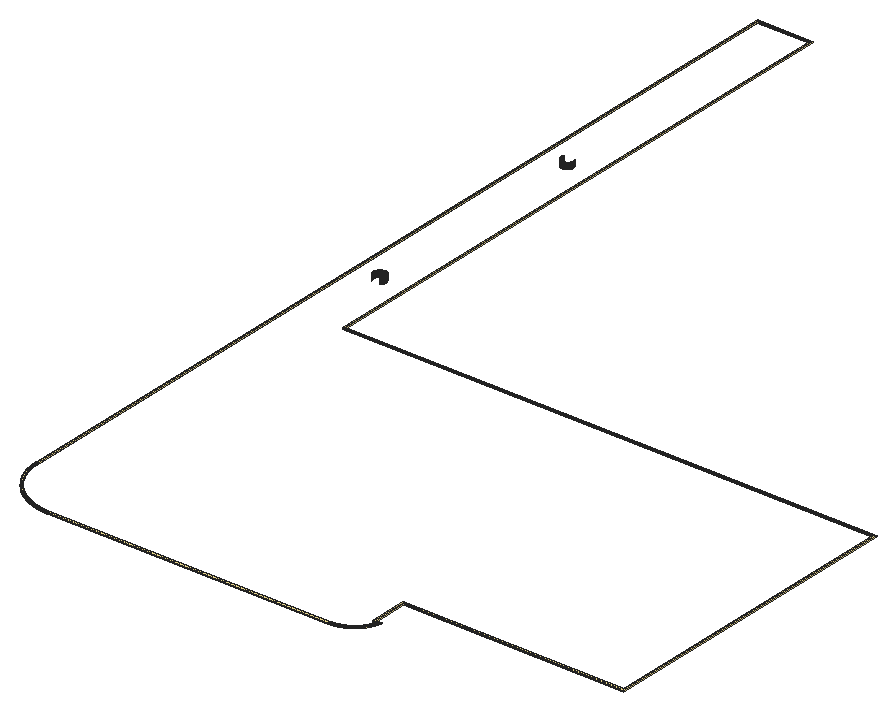
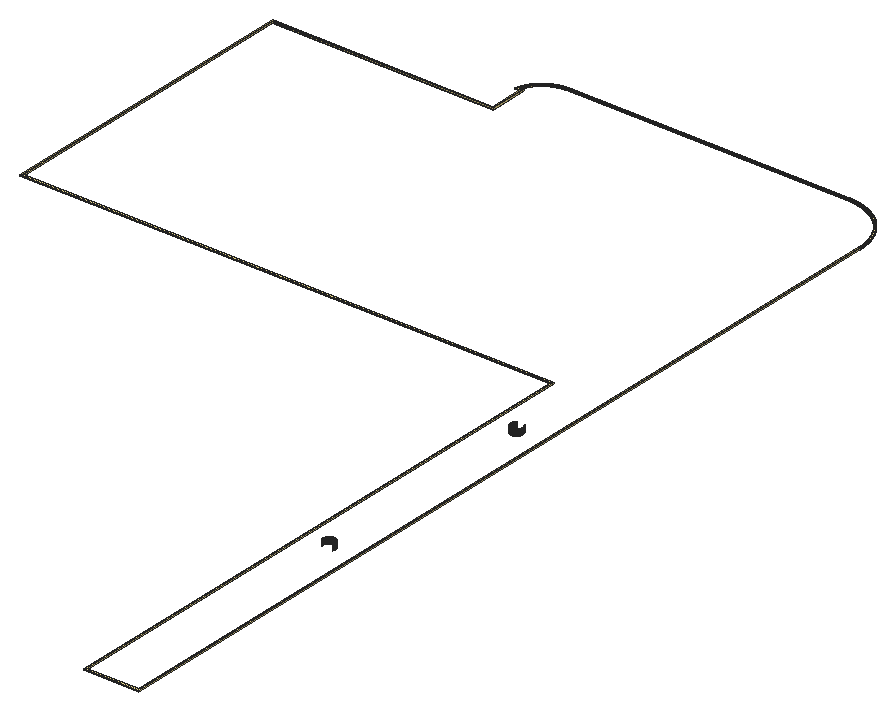
# SketchUp Ruby script. Lengths in inches.
U = 1.inch
M = Sketchup.active_model
def pt(a) = Geom::Point3d.new(a.map { |v| v * U })
def face(e, loops, mat)
  f = e.add_face(loops[0].map { |a| pt(a) })
  loops[1..].each { |l| e.add_face(l.map { |a| pt(a) }).erase! }
  f.material = f.back_material = mat if mat
  f
end
# faces: each face lists its corners as indices into pts; further lists are holes
def faces(e, pts, list, mat = nil) = list.each { |f| face(e, (f[0].is_a?(Array) ? f : [f]).map { |l| l.map { |i| pts[i] } }, mat) }
# xy, xz, yz: faces in a plane at the given z, y or x. An outline is a flat list of corners, or four numbers for a rectangle; further outlines are holes
def ring(l) = l.size == 4 ? [[l[0], l[1]], [l[2], l[1]], [l[2], l[3]], [l[0], l[3]]] : l.each_slice(2).to_a
def flat(e, list, mat, &to3) = list.each { |f| face(e, (f[0].is_a?(Array) ? f : [f]).map { |l| ring(l).map { |u, v| to3.(u, v) } }, mat) }
def xy(e, z, list, mat = nil) = flat(e, list, mat) { |x, y| [x, y, z] }
def xz(e, y, list, mat = nil) = flat(e, list, mat) { |x, z| [x, y, z] }
def yz(e, x, list, mat = nil) = flat(e, list, mat) { |y, z| [x, y, z] }
def lines(e, pts, list) = list.each { |a, b| e.add_line(pt(pts[a]), pt(pts[b])) }
# prism: a flat outline (further loops are holes) pulled along v
def prism(e, loops, v, mat = nil)
  f = face(e, loops, mat); d = Geom::Vector3d.new(v.map { |x| x * U })
  f.pushpull(f.normal.samedirection?(d) ? d.length : -d.length)
end
def box(e, o, s, mat = nil) = prism(e, [[o, [o[0] + s[0], o[1], o[2]], [o[0] + s[0], o[1] + s[1], o[2]], [o[0], o[1] + s[1], o[2]]]], [0, 0, s[2]], mat)
def at(x, y, z, deg = 0) = Geom::Transformation.translation(pt([x, y, z])) * Geom::Transformation.rotation(ORIGIN, Z_AXIS, deg.degrees)
def axes(o, x, y, z) = Geom::Transformation.new([*x, 0, *y, 0, *z, 0, *pt(o).to_a, 1])
def part(name) = M.definitions.add(name)
# library, detail: a bought-in or finely detailed component or shape, given as its bounding box
def library(name, o, s) = part(name).tap { |d| box(d.entities, o, s) }
def detail(e, o, s) = box(e.add_group.entities, o, s)
def put(e, d, t, mat = nil) = e.add_instance(d, t).tap { |i| i.material = mat if mat }
def group(e, t, mat = nil) = e.add_group.tap { |g| g.transformation = t; g.material = mat if mat }.entities
root = M.entities
M.materials.add("False Ceiling Light").color = [251, 231, 149]
xz(root,298.66,[[28.76,258,28.84,261],[29.16,258,29.24,261]])
xz(root,298.67,[[28.92,258,29,261],[29,258,29.08,261]])
xz(root,410.83,[[28.92,258,29,261],[29,258,29.08,261]])
xz(root,410.84,[[28.76,258,28.84,261],[29.16,258,29.24,261]])
yz(root,26,[[295.51,258,295.59,261],[295.59,258,295.67,261],[295.67,258,295.75,261],[295.75,258,295.82,261],[413.68,258,413.75,261],
  [413.75,258,413.83,261],[413.83,258,413.91,261],[413.91,258,413.99,261]])
yz(root,32,[[295.51,258,295.59,261],[295.59,258,295.67,261],[295.67,258,295.75,261],[295.75,258,295.82,261],[413.68,258,413.75,261],
  [413.75,258,413.83,261],[413.83,258,413.91,261],[413.91,258,413.99,261]])
p = [[26.99,293.4375,258],[26.93,293.49,258],[26.93,293.49,261],[26.99,293.4375,261],[31.07,293.49,258],[31.01,293.4375,258],
  [31.01,293.4375,261],[31.07,293.49,261],[26.88,293.55,258],[26.82,293.6,258],[26.82,293.6,261],[26.88,293.55,261],
  [31.12,293.55,258],[31.12,293.55,261],[31.18,293.6,258],[31.18,293.6,261],[26.77,293.66,258],[26.77,293.66,261],
  [31.23,293.66,258],[31.23,293.66,261],[26.72,293.72,258],[26.72,293.72,261],[26.67,293.78,258],[26.67,293.78,261],
  [31.28,293.72,258],[31.28,293.72,261],[31.33,293.78,258],[31.33,293.78,261],[26.62,293.84,258],[26.62,293.84,261],
  [26.57,293.9,258],[26.57,293.9,261],[31.38,293.84,258],[31.38,293.84,261],[31.43,293.9,258],[31.43,293.9,261],
  [26.53,293.97,258],[26.53,293.97,261],[31.47,293.97,258],[31.47,293.97,261],[26.48,294.03,258],[26.44,294.1,258],
  [26.44,294.1,261],[26.48,294.03,261],[31.52,294.03,258],[31.52,294.03,261],[31.56,294.1,258],[31.56,294.1,261],
  [26.4,294.17,258],[26.4,294.17,261],[31.6,294.17,258],[31.6,294.17,261],[26.36,294.24,258],[26.33,294.3,258],
  [26.33,294.3,261],[26.36,294.24,261],[31.64,294.24,258],[31.64,294.24,261],[31.67,294.3,258],[31.67,294.3,261],
  [26.29,294.375,258],[26.29,294.375,261],[31.71,294.375,258],[31.71,294.375,261],[26.26,294.45,258],[26.23,294.52,258],
  [26.23,294.52,261],[26.26,294.45,261],[31.74,294.45,258],[31.74,294.45,261],[31.77,294.52,258],[31.77,294.52,261],
  [26.2,294.59,258],[26.2,294.59,261],[31.8,294.59,258],[31.8,294.59,261],[26.17,294.67,258],[26.17,294.67,261],
  [31.83,294.67,258],[31.83,294.67,261],[26.15,294.74,258],[26.15,294.74,261],[26.125,294.81,258],[26.125,294.81,261],
  [31.85,294.74,258],[31.85,294.74,261],[31.875,294.81,258],[31.875,294.81,261],[26.1,294.89,258],[26.1,294.89,261],
  [31.9,294.89,258],[31.9,294.89,261],[26.08,294.97,258],[26.08,294.97,261],[31.92,294.97,258],[31.92,294.97,261],
  [26.07,295.04,258],[26.07,295.04,261],[26.05,295.12,258],[26.05,295.12,261],[31.93,295.04,258],[31.93,295.04,261],
  [31.95,295.12,258],[31.95,295.12,261],[26.04,295.2,258],[26.04,295.2,261],[31.96,295.2,258],[31.96,295.2,261],
  [26.03,295.28,258],[26.03,295.28,261],[31.97,295.28,258],[31.97,295.28,261],[26.02,295.35,258],[26.02,295.35,261],
  [31.98,295.35,258],[31.98,295.35,261],[26.01,295.43,258],[26.01,295.43,261],[26,295.51,258],[26,295.51,261],
  [31.99,295.43,258],[31.99,295.43,261],[32,295.51,258],[32,295.51,261],[26,295.82,258],[26.01,295.9,258],
  [26.01,295.9,261],[26,295.82,261],[31.99,295.9,258],[32,295.82,258],[32,295.82,261],[31.99,295.9,261],
  [26.02,295.98,258],[26.02,295.98,261],[31.98,295.98,258],[31.98,295.98,261],[26.03,296.06,258],[26.03,296.06,261],
  [31.97,296.06,258],[31.97,296.06,261],[26.04,296.14,258],[26.04,296.14,261],[26.05,296.21,258],[26.05,296.21,261],
  [31.95,296.21,258],[31.96,296.14,258],[31.96,296.14,261],[31.95,296.21,261],[26.07,296.29,258],[26.07,296.29,261],
  [31.93,296.29,258],[31.93,296.29,261],[26.08,296.37,258],[26.08,296.37,261],[31.92,296.37,258],[31.92,296.37,261],
  [26.1,296.44,258],[26.1,296.44,261],[26.125,296.52,258],[26.125,296.52,261],[31.9,296.44,258],[31.9,296.44,261],
  [31.875,296.52,258],[31.875,296.52,261],[26.15,296.59,258],[26.15,296.59,261],[31.85,296.59,258],[31.85,296.59,261],
  [26.17,296.67,258],[26.17,296.67,261],[31.83,296.67,258],[31.83,296.67,261],[26.2,296.74,258],[26.2,296.74,261],
  [26.23,296.81,258],[26.23,296.81,261],[31.8,296.74,258],[31.8,296.74,261],[31.77,296.81,258],[31.77,296.81,261],
  [26.26,296.89,258],[26.26,296.89,261],[31.74,296.89,258],[31.74,296.89,261],[26.29,296.96,258],[26.29,296.96,261],
  [31.71,296.96,258],[31.71,296.96,261],[26.33,297.03,258],[26.33,297.03,261],[26.36,297.1,258],[26.36,297.1,261],
  [31.64,297.1,258],[31.67,297.03,258],[31.67,297.03,261],[31.64,297.1,261],[26.4,297.17,258],[26.4,297.17,261],
  [31.6,297.17,258],[31.6,297.17,261],[26.44,297.23,258],[26.44,297.23,261],[26.48,297.3,258],[26.48,297.3,261],
  [31.52,297.3,258],[31.56,297.23,258],[31.56,297.23,261],[31.52,297.3,261],[26.53,297.37,258],[26.53,297.37,261],
  [31.47,297.37,258],[31.47,297.37,261],[26.57,297.43,258],[26.57,297.43,261],[26.62,297.49,258],[26.62,297.49,261],
  [31.43,297.43,258],[31.43,297.43,261],[31.38,297.49,258],[31.38,297.49,261],[26.67,297.55,258],[26.67,297.55,261],
  [31.33,297.55,258],[31.33,297.55,261],[26.72,297.62,258],[26.72,297.62,261],[26.77,297.67,258],[26.77,297.67,261],
  [31.23,297.67,258],[31.28,297.62,258],[31.28,297.62,261],[31.23,297.67,261],[26.82,297.73,258],[26.82,297.73,261],
  [26.88,297.79,258],[26.88,297.79,261],[31.12,297.79,258],[31.18,297.73,258],[31.18,297.73,261],[31.12,297.79,261],
  [26.93,297.84,258],[26.93,297.84,261],[26.99,297.9,258],[26.99,297.9,261],[31.01,297.9,258],[31.07,297.84,258],
  [31.07,297.84,261],[31.01,297.9,261],[27.05,297.95,258],[27.05,297.95,261],[27.11,298,258],[27.11,298,261],
  [30.95,297.95,258],[30.95,297.95,261],[30.89,298,258],[30.89,298,261],[27.17,298.05,258],[27.17,298.05,261],
  [27.24,298.09,258],[27.24,298.09,261],[30.83,298.05,258],[30.83,298.05,261],[30.76,298.09,258],[30.76,298.09,261],
  [27.3,298.14,258],[27.3,298.14,261],[27.37,298.18,258],[27.37,298.18,261],[30.63,298.18,258],[30.7,298.14,258],
  [30.7,298.14,261],[30.63,298.18,261],[27.43,298.22,258],[27.43,298.22,261],[27.5,298.26,258],[27.5,298.26,261],
  [30.5,298.26,258],[30.57,298.22,258],[30.57,298.22,261],[30.5,298.26,261],[27.57,298.3,258],[27.57,298.3,261],
  [27.64,298.34,258],[27.64,298.34,261],[27.71,298.375,258],[27.71,298.375,261],[30.29,298.375,258],[30.36,298.34,258],
  [30.36,298.34,261],[30.29,298.375,261],[30.43,298.3,258],[30.43,298.3,261],[27.78,298.41,258],[27.78,298.41,261],
  [27.85,298.4375,258],[27.85,298.4375,261],[27.92,298.47,258],[27.92,298.47,261],[30.15,298.4375,258],[30.22,298.41,258],
  [30.22,298.41,261],[30.15,298.4375,261],[30.08,298.47,258],[30.08,298.47,261],[28,298.49,258],[28,298.49,261],
  [28.07,298.52,258],[28.07,298.52,261],[28.15,298.54,258],[28.15,298.54,261],[28.22,298.5625,258],[28.22,298.5625,261],
  [29.78,298.5625,258],[29.85,298.54,258],[29.85,298.54,261],[29.78,298.5625,261],[29.93,298.52,258],[30,298.49,258],
  [30,298.49,261],[29.93,298.52,261],[28.3,298.58,258],[28.3,298.58,261],[28.375,298.6,258],[28.375,298.6,261],
  [28.45,298.62,258],[28.45,298.62,261],[28.53,298.63,258],[28.53,298.63,261],[28.61,298.64,258],[28.61,298.64,261],
  [28.6875,298.65,258],[28.6875,298.65,261],[29.3125,298.65,258],[29.39,298.64,258],[29.39,298.64,261],[29.3125,298.65,261],
  [29.47,298.63,258],[29.47,298.63,261],[29.55,298.62,258],[29.625,298.6,258],[29.625,298.6,261],[29.55,298.62,261],
  [29.7,298.58,258],[29.7,298.58,261],[28.76,298.66,258],[28.76,298.66,261],[28.84,298.66,258],[28.92,298.67,258],
  [28.92,298.67,261],[28.84,298.66,261],[29.08,298.67,258],[29.16,298.66,258],[29.16,298.66,261],[29.08,298.67,261],
  [29.24,298.66,258],[29.24,298.66,261],[28.6875,410.85,258],[28.61,410.86,258],[28.61,410.86,261],[28.6875,410.85,261],
  [28.76,410.84,258],[28.76,410.84,261],[28.92,410.83,258],[28.84,410.84,258],[28.84,410.84,261],[28.92,410.83,261],
  [29.16,410.84,258],[29.08,410.83,258],[29.08,410.83,261],[29.16,410.84,261],[29.3125,410.85,258],[29.24,410.84,258],
  [29.24,410.84,261],[29.3125,410.85,261],[29.39,410.86,258],[29.39,410.86,261],[28.22,410.9375,258],[28.15,410.96,258],
  [28.15,410.96,261],[28.22,410.9375,261],[28.3,410.92,258],[28.3,410.92,261],[28.375,410.9,258],[28.375,410.9,261],
  [28.45,410.88,258],[28.45,410.88,261],[28.53,410.87,258],[28.53,410.87,261],[29.47,410.87,258],[29.47,410.87,261],
  [29.55,410.88,258],[29.55,410.88,261],[29.625,410.9,258],[29.625,410.9,261],[29.7,410.92,258],[29.7,410.92,261],
  [29.78,410.9375,258],[29.78,410.9375,261],[29.85,410.96,258],[29.85,410.96,261],[28,411.01,258],[27.92,411.03,258],
  [27.92,411.03,261],[28,411.01,261],[27.85,411.0625,258],[27.85,411.0625,261],[28.07,410.98,258],[28.07,410.98,261],
  [29.93,410.98,258],[29.93,410.98,261],[30,411.01,258],[30,411.01,261],[30.08,411.03,258],[30.08,411.03,261],
  [30.15,411.0625,258],[30.15,411.0625,261],[27.71,411.125,258],[27.64,411.16,258],[27.64,411.16,261],[27.71,411.125,261],
  [27.78,411.09,258],[27.78,411.09,261],[30.22,411.09,258],[30.22,411.09,261],[30.29,411.125,258],[30.29,411.125,261],
  [30.36,411.16,258],[30.36,411.16,261],[27.5,411.24,258],[27.43,411.28,258],[27.43,411.28,261],[27.5,411.24,261],
  [27.57,411.2,258],[27.57,411.2,261],[30.43,411.2,258],[30.43,411.2,261],[30.5,411.24,258],[30.5,411.24,261],
  [30.57,411.28,258],[30.57,411.28,261],[27.37,411.32,258],[27.3,411.36,258],[27.3,411.36,261],[27.37,411.32,261],
  [30.63,411.32,258],[30.63,411.32,261],[30.7,411.36,258],[30.7,411.36,261],[27.24,411.41,258],[27.24,411.41,261],
  [27.17,411.45,258],[27.17,411.45,261],[30.76,411.41,258],[30.76,411.41,261],[30.83,411.45,258],[30.83,411.45,261],
  [27.11,411.5,258],[27.11,411.5,261],[27.05,411.55,258],[27.05,411.55,261],[30.89,411.5,258],[30.89,411.5,261],
  [30.95,411.55,258],[30.95,411.55,261],[26.99,411.6,258],[26.93,411.66,258],[26.93,411.66,261],[26.99,411.6,261],
  [31.01,411.6,258],[31.01,411.6,261],[31.07,411.66,258],[31.07,411.66,261],[26.88,411.71,258],[26.82,411.77,258],
  [26.82,411.77,261],[26.88,411.71,261],[31.12,411.71,258],[31.12,411.71,261],[31.18,411.77,258],[31.18,411.77,261],
  [26.77,411.83,258],[26.72,411.88,258],[26.72,411.88,261],[26.77,411.83,261],[31.23,411.83,258],[31.23,411.83,261],
  [31.28,411.88,258],[31.28,411.88,261],[26.67,411.95,258],[26.62,412.01,258],[26.62,412.01,261],[26.67,411.95,261],
  [31.33,411.95,258],[31.33,411.95,261],[31.38,412.01,258],[31.38,412.01,261],[26.57,412.07,258],[26.57,412.07,261],
  [31.43,412.07,258],[31.43,412.07,261],[26.53,412.13,258],[26.53,412.13,261],[26.48,412.2,258],[26.48,412.2,261],
  [31.47,412.13,258],[31.47,412.13,261],[31.52,412.2,258],[31.52,412.2,261],[26.44,412.27,258],[26.44,412.27,261],
  [31.56,412.27,258],[31.56,412.27,261],[26.4,412.33,258],[26.4,412.33,261],[26.36,412.4,258],[26.36,412.4,261],
  [31.6,412.33,258],[31.6,412.33,261],[31.64,412.4,258],[31.64,412.4,261],[26.33,412.47,258],[26.33,412.47,261],
  [31.67,412.47,258],[31.67,412.47,261],[26.29,412.54,258],[26.29,412.54,261],[26.26,412.61,258],[26.26,412.61,261],
  [31.71,412.54,258],[31.71,412.54,261],[31.74,412.61,258],[31.74,412.61,261],[26.23,412.69,258],[26.23,412.69,261],
  [31.77,412.69,258],[31.77,412.69,261],[26.2,412.76,258],[26.2,412.76,261],[31.8,412.76,258],[31.8,412.76,261],
  [26.17,412.83,258],[26.15,412.91,258],[26.15,412.91,261],[26.17,412.83,261],[31.83,412.83,258],[31.83,412.83,261],
  [31.85,412.91,258],[31.85,412.91,261],[26.125,412.98,258],[26.125,412.98,261],[31.875,412.98,258],[31.875,412.98,261],
  [26.1,413.06,258],[26.1,413.06,261],[31.9,413.06,258],[31.9,413.06,261],[26.08,413.13,258],[26.08,413.13,261],
  [26.07,413.21,258],[26.07,413.21,261],[31.92,413.13,258],[31.92,413.13,261],[31.93,413.21,258],[31.93,413.21,261],
  [26.05,413.29,258],[26.05,413.29,261],[31.95,413.29,258],[31.95,413.29,261],[26.04,413.36,258],[26.04,413.36,261],
  [31.96,413.36,258],[31.96,413.36,261],[26.03,413.44,258],[26.03,413.44,261],[26.02,413.52,258],[26.02,413.52,261],
  [31.97,413.44,258],[31.97,413.44,261],[31.98,413.52,258],[31.98,413.52,261],[26.01,413.6,258],[26.01,413.6,261],
  [31.99,413.6,258],[31.99,413.6,261],[26,413.68,258],[26,413.68,261],[32,413.68,258],[32,413.68,261],
  [26,413.99,258],[26.01,414.07,258],[26.01,414.07,261],[26,413.99,261],[31.99,414.07,258],[32,413.99,258],
  [32,413.99,261],[31.99,414.07,261],[26.02,414.15,258],[26.02,414.15,261],[26.03,414.22,258],[26.03,414.22,261],
  [31.98,414.15,258],[31.98,414.15,261],[31.97,414.22,258],[31.97,414.22,261],[26.04,414.3,258],[26.04,414.3,261],
  [31.96,414.3,258],[31.96,414.3,261],[26.05,414.38,258],[26.05,414.38,261],[31.95,414.38,258],[31.95,414.38,261],
  [26.07,414.46,258],[26.07,414.46,261],[31.93,414.46,258],[31.93,414.46,261],[26.08,414.53,258],[26.08,414.53,261],
  [26.1,414.61,258],[26.1,414.61,261],[31.92,414.53,258],[31.92,414.53,261],[31.9,414.61,258],[31.9,414.61,261],
  [26.125,414.69,258],[26.125,414.69,261],[31.875,414.69,258],[31.875,414.69,261],[26.15,414.76,258],[26.15,414.76,261],
  [31.85,414.76,258],[31.85,414.76,261],[26.17,414.83,258],[26.17,414.83,261],[26.2,414.91,258],[26.2,414.91,261],
  [31.83,414.83,258],[31.83,414.83,261]]
faces(root,p,[[0,1,2,3],[4,5,6,7],[8,9,10,11],[1,8,11,2],[12,4,7,13],[14,12,13,15],[9,16,17,10],[18,14,15,19],
  [16,20,21,17],[20,22,23,21],[24,18,19,25],[26,24,25,27],[22,28,29,23],[28,30,31,29],[32,26,27,33],[34,32,33,35],
  [30,36,37,31],[38,34,35,39],[40,41,42,43],[36,40,43,37],[44,38,39,45],[46,44,45,47],[41,48,49,42],[50,46,47,51],
  [52,53,54,55],[48,52,55,49],[56,50,51,57],[58,56,57,59],[53,60,61,54],[62,58,59,63],[64,65,66,67],[60,64,67,61],
  [68,62,63,69],[70,68,69,71],[65,72,73,66],[74,70,71,75],[72,76,77,73],[78,74,75,79],[76,80,81,77],[80,82,83,81],
  [84,78,79,85],[86,84,85,87],[82,88,89,83],[90,86,87,91],[88,92,93,89],[94,90,91,95],[92,96,97,93],[96,98,99,97],
  [100,94,95,101],[102,100,101,103],[98,104,105,99],[106,102,103,107],[104,108,109,105],[110,106,107,111],[108,112,113,109],[114,110,111,115],
  [112,116,117,113],[116,118,119,117],[120,114,115,121],[122,120,121,123],[124,125,126,127],[128,129,130,131],[125,132,133,126],[134,128,131,135],
  [132,136,137,133],[138,134,135,139],[136,140,141,137],[140,142,143,141],[144,145,146,147],[145,138,139,146],[142,148,149,143],[150,144,147,151],
  [148,152,153,149],[154,150,151,155],[152,156,157,153],[156,158,159,157],[160,154,155,161],[162,160,161,163],[158,164,165,159],[166,162,163,167],
  [164,168,169,165],[170,166,167,171],[168,172,173,169],[172,174,175,173],[176,170,171,177],[178,176,177,179],[174,180,181,175],[182,178,179,183],
  [180,184,185,181],[186,182,183,187],[184,188,189,185],[188,190,191,189],[192,193,194,195],[193,186,187,194],[190,196,197,191],[198,192,195,199],
  [196,200,201,197],[200,202,203,201],[204,205,206,207],[205,198,199,206],[202,208,209,203],[210,204,207,211],[208,212,213,209],[212,214,215,213],
  [216,210,211,217],[218,216,217,219],[214,220,221,215],[222,218,219,223],[220,224,225,221],[224,226,227,225],[228,229,230,231],[229,222,223,230],
  [226,232,233,227],[232,234,235,233],[236,237,238,239],[237,228,231,238],[234,240,241,235],[240,242,243,241],[244,245,246,247],[245,236,239,246],
  [242,248,249,243],[248,250,251,249],[252,244,247,253],[254,252,253,255],[250,256,257,251],[256,258,259,257],[260,254,255,261],[262,260,261,263],
  [258,264,265,259],[264,266,267,265],[268,269,270,271],[269,262,263,270],[266,272,273,267],[272,274,275,273],[276,277,278,279],[277,268,271,278],
  [274,280,281,275],[280,282,283,281],[282,284,285,283],[286,287,288,289],[290,276,279,291],[287,290,291,288],[284,292,293,285],[292,294,295,293],
  [294,296,297,295],[298,299,300,301],[302,298,301,303],[299,286,289,300],[296,304,305,297],[304,306,307,305],[306,308,309,307],[308,310,311,309],
  [312,313,314,315],[316,317,318,319],[313,316,319,314],[317,302,303,318],[310,320,321,311],[320,322,323,321],[322,324,325,323],[324,326,327,325],
  [326,328,329,327],[328,330,331,329],[332,333,334,335],[333,336,337,334],[338,339,340,341],[336,338,341,337],[339,342,343,340],[342,312,315,343],
  [330,344,345,331],[346,347,348,349],[350,351,352,353],[354,332,335,355],[356,357,358,359],[360,356,359,361],[362,363,364,365],[366,367,368,369],
  [370,371,372,373],[374,370,373,375],[376,377,378,379],[380,376,379,381],[382,380,381,383],[384,382,383,385],[357,386,387,358],[386,384,385,387],
  [388,374,375,389],[390,388,389,391],[392,390,391,393],[394,392,393,395],[396,394,395,397],[398,396,397,399],[400,401,402,403],[401,404,405,402],
  [406,400,403,407],[377,406,407,378],[408,398,399,409],[410,408,409,411],[412,410,411,413],[414,412,413,415],[416,417,418,419],[420,416,419,421],
  [404,420,421,405],[422,414,415,423],[424,422,423,425],[426,424,425,427],[428,429,430,431],[432,428,431,433],[417,432,433,418],[434,426,427,435],
  [436,434,435,437],[438,436,437,439],[440,441,442,443],[429,440,443,430],[444,438,439,445],[446,444,445,447],[441,448,449,442],[448,450,451,449],
  [452,446,447,453],[454,452,453,455],[450,456,457,451],[456,458,459,457],[460,454,455,461],[462,460,461,463],[464,465,466,467],[458,464,467,459],
  [468,462,463,469],[470,468,469,471],[472,473,474,475],[465,472,475,466],[476,470,471,477],[478,476,477,479],[480,481,482,483],[473,480,483,474],
  [484,478,479,485],[486,484,485,487],[488,489,490,491],[481,488,491,482],[492,486,487,493],[494,492,493,495],[489,496,497,490],[498,494,495,499],
  [496,500,501,497],[500,502,503,501],[504,498,499,505],[506,504,505,507],[502,508,509,503],[510,506,507,511],[508,512,513,509],[512,514,515,513],
  [516,510,511,517],[518,516,517,519],[514,520,521,515],[522,518,519,523],[520,524,525,521],[524,526,527,525],[528,522,523,529],[530,528,529,531],
  [526,532,533,527],[534,530,531,535],[532,536,537,533],[538,534,535,539],[540,541,542,543],[536,540,543,537],[544,538,539,545],[546,544,545,547],
  [541,548,549,542],[550,546,547,551],[548,552,553,549],[554,550,551,555],[552,556,557,553],[556,558,559,557],[560,554,555,561],[562,560,561,563],
  [558,564,565,559],[566,562,563,567],[564,568,569,565],[570,566,567,571],[568,572,573,569],[572,574,575,573],[576,570,571,577],[578,576,577,579],
  [574,580,581,575],[582,578,579,583],[580,584,585,581],[586,582,583,587],[588,589,590,591],[592,593,594,595],[589,596,597,590],[596,598,599,597],
  [600,592,595,601],[602,600,601,603],[598,604,605,599],[606,602,603,607],[604,608,609,605],[610,606,607,611],[608,612,613,609],[614,610,611,615],
  [612,616,617,613],[616,618,619,617],[620,614,615,621],[622,620,621,623],[618,624,625,619],[626,622,623,627],[624,628,629,625],[630,626,627,631],
  [628,632,633,629],[632,634,635,633],[636,630,631,637]])
g1 = group(root,at(15,68,258.5),"False Ceiling Light")
prism(g1,[[[0,483,-0.5],[28,483,-0.5],[28,189,-0.5],[295,189,-0.5],[295,30,-0.5],[184,30,-0.5],[184,13,-0.5],[186.52,13,-0.5],[186.48,12.82,-0.5],[186.42,12.6,-0.5],[186.36,12.39,-0.5],[186.3,12.17,-0.5],[186.24,11.96,-0.5],[186.17,11.75,-0.5],[186.1,11.54,-0.5],[186.02,11.33,-0.5],[185.95,11.12,-0.5],[185.87,10.91,-0.5],[185.79,10.7,-0.5],[185.71,10.49,-0.5],[185.62,10.29,-0.5],[185.53,10.09,-0.5],[185.4375,9.88,-0.5],[185.34,9.68,-0.5],[185.25,9.48,-0.5],[185.15,9.28,-0.5],[185.04,9.08,-0.5],[184.94,8.89,-0.5],[184.83,8.69,-0.5],[184.72,8.5,-0.5],[184.61,8.31,-0.5],[184.49,8.12,-0.5],[184.38,7.93,-0.5],[184.26,7.74,-0.5],[184.13,7.56,-0.5],[184.01,7.37,-0.5],[183.88,7.1875,-0.5],[183.75,7.01,-0.5],[183.62,6.83,-0.5],[183.49,6.65,-0.5],[183.35,6.48,-0.5],[183.21,6.3,-0.5],[183.07,6.13,-0.5],[182.93,5.96,-0.5],[182.78,5.79,-0.5],[182.63,5.625,-0.5],[182.48,5.46,-0.5],[182.33,5.3,-0.5],[182.18,5.14,-0.5],[182.02,4.98,-0.5],[181.86,4.82,-0.5],[181.7,4.67,-0.5],[181.54,4.52,-0.5],[181.375,4.37,-0.5],[181.21,4.22,-0.5],[181.04,4.07,-0.5],[180.87,3.93,-0.5],[180.7,3.79,-0.5],[180.52,3.65,-0.5],[180.35,3.51,-0.5],[180.17,3.38,-0.5],[179.99,3.25,-0.5],[179.8125,3.12,-0.5],[179.63,2.99,-0.5],[179.44,2.87,-0.5],[179.26,2.74,-0.5],[179.07,2.62,-0.5],[178.88,2.51,-0.5],[178.69,2.39,-0.5],[178.5,2.28,-0.5],[178.31,2.17,-0.5],[178.11,2.06,-0.5],[177.92,1.96,-0.5],[177.72,1.85,-0.5],[177.52,1.75,-0.5],[177.32,1.66,-0.5],[177.12,1.5625,-0.5],[176.91,1.47,-0.5],[176.71,1.38,-0.5],[176.51,1.29,-0.5],[176.3,1.21,-0.5],[176.09,1.13,-0.5],[175.88,1.05,-0.5],[175.67,0.98,-0.5],[175.46,0.9,-0.5],[175.25,0.83,-0.5],[175.04,0.76,-0.5],[174.83,0.7,-0.5],[174.61,0.64,-0.5],[174.4,0.58,-0.5],[174.18,0.52,-0.5],[173.97,0.47,-0.5],[173.75,0.42,-0.5],[173.53,0.37,-0.5],[173.32,0.33,-0.5],[173.1,0.28,-0.5],[172.88,0.25,-0.5],[172.66,0.21,-0.5],[172.4375,0.18,-0.5],[172.22,0.15,-0.5],[172,0.12,-0.5],[171.78,0.09,-0.5],[171.56,0.07,-0.5],[171.33,0.05,-0.5],[171.11,0.04,-0.5],[170.89,0.02,-0.5],[170.67,0.01,-0.5],[170.45,0.01,-0.5],[170.22,0,-0.5],[169.99,0,-0.5],[29,0,-0.5],[28.62,0,-0.5],[28.24,0.01,-0.5],[27.86,0.02,-0.5],[27.48,0.04,-0.5],[27.1,0.0625,-0.5],[26.72,0.09,-0.5],[26.35,0.12,-0.5],[25.97,0.16,-0.5],[25.59,0.2,-0.5],[25.21,0.25,-0.5],[24.84,0.3,-0.5],[24.46,0.36,-0.5],[24.09,0.42,-0.5],[23.72,0.49,-0.5],[23.34,0.56,-0.5],[22.97,0.63,-0.5],[22.6,0.72,-0.5],[22.23,0.8,-0.5],[21.86,0.89,-0.5],[21.49,0.99,-0.5],[21.13,1.09,-0.5],[20.76,1.19,-0.5],[20.4,1.3,-0.5],[20.04,1.42,-0.5],[19.68,1.54,-0.5],[19.32,1.66,-0.5],[18.96,1.79,-0.5],[18.61,1.93,-0.5],[18.25,2.06,-0.5],[17.9,2.21,-0.5],[17.55,2.36,-0.5],[17.2,2.51,-0.5],[16.86,2.66,-0.5],[16.52,2.83,-0.5],[16.17,2.99,-0.5],[15.83,3.16,-0.5],[15.5,3.34,-0.5],[15.16,3.51,-0.5],[14.83,3.7,-0.5],[14.5,3.89,-0.5],[14.17,4.08,-0.5],[13.85,4.27,-0.5],[13.53,4.47,-0.5],[13.21,4.68,-0.5],[12.89,4.89,-0.5],[12.57,5.1,-0.5],[12.26,5.32,-0.5],[11.95,5.54,-0.5],[11.65,5.76,-0.5],[11.35,5.99,-0.5],[11.05,6.23,-0.5],[10.75,6.46,-0.5],[10.46,6.7,-0.5],[10.17,6.95,-0.5],[9.88,7.2,-0.5],[9.6,7.45,-0.5],[9.31,7.7,-0.5],[9.04,7.96,-0.5],[8.76,8.23,-0.5],[8.49,8.49,-0.5],[8.23,8.76,-0.5],[7.96,9.04,-0.5],[7.7,9.31,-0.5],[7.45,9.6,-0.5],[7.2,9.88,-0.5],[6.95,10.17,-0.5],[6.7,10.46,-0.5],[6.46,10.75,-0.5],[6.23,11.05,-0.5],[5.99,11.35,-0.5],[5.76,11.65,-0.5],[5.54,11.95,-0.5],[5.32,12.26,-0.5],[5.1,12.57,-0.5],[4.89,12.89,-0.5],[4.68,13.21,-0.5],[4.47,13.53,-0.5],[4.27,13.85,-0.5],[4.08,14.17,-0.5],[3.89,14.5,-0.5],[3.7,14.83,-0.5],[3.51,15.16,-0.5],[3.34,15.5,-0.5],[3.16,15.83,-0.5],[2.99,16.17,-0.5],[2.83,16.52,-0.5],[2.66,16.86,-0.5],[2.51,17.2,-0.5],[2.36,17.55,-0.5],[2.21,17.9,-0.5],[2.06,18.25,-0.5],[1.93,18.61,-0.5],[1.79,18.96,-0.5],[1.66,19.32,-0.5],[1.54,19.68,-0.5],[1.42,20.04,-0.5],[1.3,20.4,-0.5],[1.19,20.76,-0.5],[1.09,21.13,-0.5],[0.99,21.49,-0.5],[0.89,21.86,-0.5],[0.8,22.23,-0.5],[0.72,22.6,-0.5],[0.63,22.97,-0.5],[0.56,23.34,-0.5],[0.49,23.72,-0.5],[0.42,24.09,-0.5],[0.36,24.46,-0.5],[0.3,24.84,-0.5],[0.25,25.21,-0.5],[0.2,25.59,-0.5],[0.16,25.97,-0.5],[0.12,26.35,-0.5],[0.09,26.72,-0.5],[0.0625,27.1,-0.5],[0.04,27.48,-0.5],[0.02,27.86,-0.5],[0.01,28.24,-0.5],[0,28.62,-0.5],[0,29,-0.5]],[[183.86,9,-0.5],[183.96,9.18,-0.5],[184.0625,9.37,-0.5],[184.16,9.55,-0.5],[184.26,9.74,-0.5],[184.35,9.92,-0.5],[184.44,10.11,-0.5],[184.53,10.3,-0.5],[184.62,10.49,-0.5],[184.7,10.68,-0.5],[184.78,10.88,-0.5],[184.86,11.07,-0.5],[184.9375,11.27,-0.5],[185.01,11.46,-0.5],[185.08,11.66,-0.5],[185.15,11.86,-0.5],[185.2,12,-0.5],[183,12,-0.5],[183,31,-0.5],[294,31,-0.5],[294,188,-0.5],[27,188,-0.5],[27,482,-0.5],[1,482,-0.5],[1,29,-0.5],[1,28.63,-0.5],[1.01,28.27,-0.5],[1.02,27.9,-0.5],[1.04,27.53,-0.5],[1.06,27.17,-0.5],[1.09,26.8,-0.5],[1.12,26.4375,-0.5],[1.15,26.07,-0.5],[1.19,25.71,-0.5],[1.24,25.35,-0.5],[1.29,24.98,-0.5],[1.34,24.62,-0.5],[1.4,24.26,-0.5],[1.47,23.9,-0.5],[1.54,23.54,-0.5],[1.61,23.18,-0.5],[1.69,22.82,-0.5],[1.77,22.46,-0.5],[1.86,22.11,-0.5],[1.95,21.75,-0.5],[2.05,21.4,-0.5],[2.15,21.05,-0.5],[2.26,20.7,-0.5],[2.37,20.35,-0.5],[2.49,20,-0.5],[2.61,19.65,-0.5],[2.73,19.31,-0.5],[2.86,18.97,-0.5],[2.99,18.625,-0.5],[3.13,18.28,-0.5],[3.27,17.95,-0.5],[3.42,17.61,-0.5],[3.57,17.28,-0.5],[3.73,16.95,-0.5],[3.89,16.62,-0.5],[4.05,16.29,-0.5],[4.22,15.96,-0.5],[4.39,15.64,-0.5],[4.57,15.32,-0.5],[4.75,15,-0.5],[4.9375,14.68,-0.5],[5.125,14.37,-0.5],[5.32,14.06,-0.5],[5.52,13.75,-0.5],[5.72,13.44,-0.5],[5.92,13.14,-0.5],[6.13,12.84,-0.5],[6.35,12.54,-0.5],[6.56,12.25,-0.5],[6.79,11.95,-0.5],[7.01,11.67,-0.5],[7.24,11.38,-0.5],[7.47,11.1,-0.5],[7.71,10.82,-0.5],[7.95,10.54,-0.5],[8.19,10.26,-0.5],[8.4375,9.99,-0.5],[8.69,9.73,-0.5],[8.94,9.46,-0.5],[9.2,9.2,-0.5],[9.46,8.94,-0.5],[9.73,8.69,-0.5],[9.99,8.4375,-0.5],[10.26,8.19,-0.5],[10.54,7.95,-0.5],[10.82,7.71,-0.5],[11.1,7.47,-0.5],[11.38,7.24,-0.5],[11.67,7.01,-0.5],[11.95,6.79,-0.5],[12.25,6.56,-0.5],[12.54,6.35,-0.5],[12.84,6.13,-0.5],[13.14,5.92,-0.5],[13.44,5.72,-0.5],[13.75,5.52,-0.5],[14.06,5.32,-0.5],[14.37,5.125,-0.5],[14.68,4.9375,-0.5],[15,4.75,-0.5],[15.32,4.57,-0.5],[15.64,4.39,-0.5],[15.96,4.22,-0.5],[16.29,4.05,-0.5],[16.62,3.89,-0.5],[16.95,3.73,-0.5],[17.28,3.57,-0.5],[17.61,3.42,-0.5],[17.95,3.27,-0.5],[18.28,3.13,-0.5],[18.625,2.99,-0.5],[18.97,2.86,-0.5],[19.31,2.73,-0.5],[19.65,2.61,-0.5],[20,2.49,-0.5],[20.35,2.37,-0.5],[20.7,2.26,-0.5],[21.05,2.15,-0.5],[21.4,2.05,-0.5],[21.75,1.95,-0.5],[22.11,1.86,-0.5],[22.46,1.77,-0.5],[22.82,1.69,-0.5],[23.18,1.61,-0.5],[23.54,1.54,-0.5],[23.9,1.47,-0.5],[24.26,1.4,-0.5],[24.62,1.34,-0.5],[24.98,1.29,-0.5],[25.35,1.24,-0.5],[25.71,1.19,-0.5],[26.07,1.15,-0.5],[26.4375,1.12,-0.5],[26.8,1.09,-0.5],[27.17,1.06,-0.5],[27.53,1.04,-0.5],[27.9,1.02,-0.5],[28.27,1.01,-0.5],[28.63,1,-0.5],[29,1,-0.5],[169.98,1,-0.5],[170.21,1,-0.5],[170.42,1.01,-0.5],[170.63,1.01,-0.5],[170.84,1.02,-0.5],[171.05,1.03,-0.5],[171.26,1.05,-0.5],[171.46,1.07,-0.5],[171.67,1.09,-0.5],[171.88,1.11,-0.5],[172.09,1.14,-0.5],[172.3,1.17,-0.5],[172.5,1.2,-0.5],[172.71,1.23,-0.5],[172.92,1.27,-0.5],[173.12,1.31,-0.5],[173.33,1.35,-0.5],[173.53,1.39,-0.5],[173.74,1.44,-0.5],[173.9375,1.49,-0.5],[174.14,1.55,-0.5],[174.34,1.6,-0.5],[174.54,1.66,-0.5],[174.74,1.72,-0.5],[174.94,1.78,-0.5],[175.14,1.85,-0.5],[175.34,1.92,-0.5],[175.54,1.99,-0.5],[175.73,2.0625,-0.5],[175.93,2.14,-0.5],[176.12,2.22,-0.5],[176.32,2.3,-0.5],[176.51,2.38,-0.5],[176.7,2.47,-0.5],[176.89,2.56,-0.5],[177.08,2.65,-0.5],[177.26,2.74,-0.5],[177.45,2.84,-0.5],[177.63,2.9375,-0.5],[177.82,3.04,-0.5],[178,3.14,-0.5],[178.18,3.25,-0.5],[178.36,3.36,-0.5],[178.54,3.47,-0.5],[178.71,3.58,-0.5],[178.89,3.7,-0.5],[179.0625,3.8125,-0.5],[179.23,3.93,-0.5],[179.4,4.06,-0.5],[179.57,4.18,-0.5],[179.74,4.31,-0.5],[179.91,4.44,-0.5],[180.07,4.57,-0.5],[180.23,4.7,-0.5],[180.39,4.83,-0.5],[180.55,4.97,-0.5],[180.71,5.11,-0.5],[180.86,5.25,-0.5],[181.01,5.39,-0.5],[181.16,5.54,-0.5],[181.3125,5.6875,-0.5],[181.46,5.84,-0.5],[181.61,5.99,-0.5],[181.75,6.14,-0.5],[181.89,6.29,-0.5],[182.03,6.45,-0.5],[182.17,6.61,-0.5],[182.3,6.77,-0.5],[182.43,6.93,-0.5],[182.56,7.09,-0.5],[182.69,7.26,-0.5],[182.82,7.43,-0.5],[182.94,7.6,-0.5],[183.07,7.77,-0.5],[183.1875,7.9375,-0.5],[183.3,8.11,-0.5],[183.42,8.29,-0.5],[183.53,8.46,-0.5],[183.64,8.64,-0.5],[183.75,8.82,-0.5]]],[0,0,0.5])
